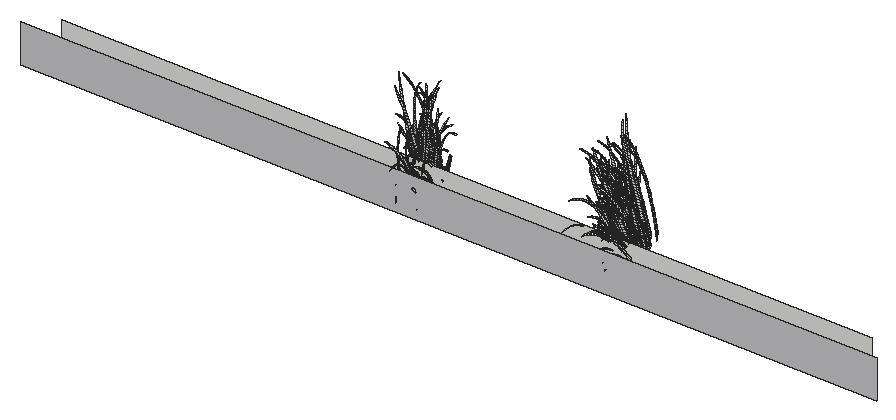
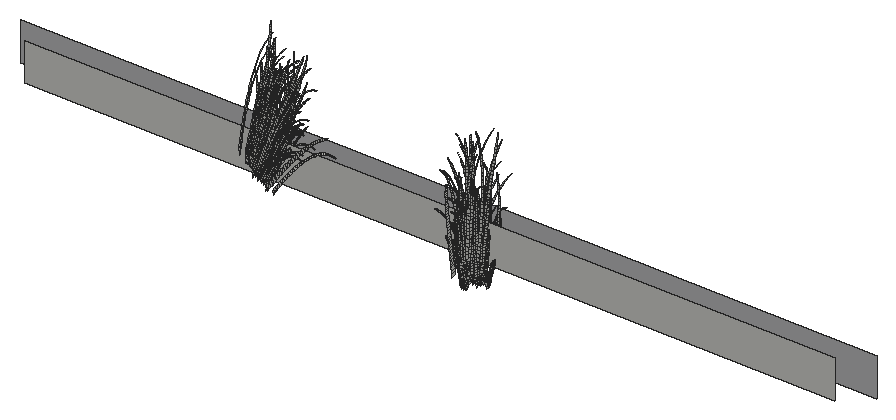
# SketchUp Ruby script. Lengths in inches.
U = 1.inch
M = Sketchup.active_model
def pt(a) = Geom::Point3d.new(a.map { |v| v * U })
def face(e, loops, mat)
  f = e.add_face(loops[0].map { |a| pt(a) })
  loops[1..].each { |l| e.add_face(l.map { |a| pt(a) }).erase! }
  f.material = f.back_material = mat if mat
  f
end
# faces: each face lists its corners as indices into pts; further lists are holes
def faces(e, pts, list, mat = nil) = list.each { |f| face(e, (f[0].is_a?(Array) ? f : [f]).map { |l| l.map { |i| pts[i] } }, mat) }
# xy, xz, yz: faces in a plane at the given z, y or x. An outline is a flat list of corners, or four numbers for a rectangle; further outlines are holes
def ring(l) = l.size == 4 ? [[l[0], l[1]], [l[2], l[1]], [l[2], l[3]], [l[0], l[3]]] : l.each_slice(2).to_a
def flat(e, list, mat, &to3) = list.each { |f| face(e, (f[0].is_a?(Array) ? f : [f]).map { |l| ring(l).map { |u, v| to3.(u, v) } }, mat) }
def xy(e, z, list, mat = nil) = flat(e, list, mat) { |x, y| [x, y, z] }
def xz(e, y, list, mat = nil) = flat(e, list, mat) { |x, z| [x, y, z] }
def yz(e, x, list, mat = nil) = flat(e, list, mat) { |y, z| [x, y, z] }
def lines(e, pts, list) = list.each { |a, b| e.add_line(pt(pts[a]), pt(pts[b])) }
# prism: a flat outline (further loops are holes) pulled along v
def prism(e, loops, v, mat = nil)
  f = face(e, loops, mat); d = Geom::Vector3d.new(v.map { |x| x * U })
  f.pushpull(f.normal.samedirection?(d) ? d.length : -d.length)
end
def box(e, o, s, mat = nil) = prism(e, [[o, [o[0] + s[0], o[1], o[2]], [o[0] + s[0], o[1] + s[1], o[2]], [o[0], o[1] + s[1], o[2]]]], [0, 0, s[2]], mat)
def at(x, y, z, deg = 0) = Geom::Transformation.translation(pt([x, y, z])) * Geom::Transformation.rotation(ORIGIN, Z_AXIS, deg.degrees)
def axes(o, x, y, z) = Geom::Transformation.new([*x, 0, *y, 0, *z, 0, *pt(o).to_a, 1])
def part(name) = M.definitions.add(name)
# library, detail: a bought-in or finely detailed component or shape, given as its bounding box
def library(name, o, s) = part(name).tap { |d| box(d.entities, o, s) }
def detail(e, o, s) = box(e.add_group.entities, o, s)
def put(e, d, t, mat = nil) = e.add_instance(d, t).tap { |i| i.material = mat if mat }
def group(e, t, mat = nil) = e.add_group.tap { |g| g.transformation = t; g.material = mat if mat }.entities
root = M.entities
M.materials.add("[Polished Concrete New]").color = [200, 200, 203]
c1 = part("fur_instance\#8")
p = [[-0.25,1.49,0.03],[0.25,-1.49,-0.03],[0.44,-1.47,1.51],[-0.05,1.47,1.57],[0.65,-1.44,3.05],[0.16,1.45,3.11],
  [0.86,-1.42,4.59],[0.38,1.44,4.65],[1.1,-1.39,6.13],[0.62,1.43,6.18],[1.34,-1.35,7.66],[0.875,1.42,7.72],
  [1.6,-1.32,9.19],[1.14,1.41,9.25],[1.88,-1.28,10.72],[1.43,1.41,10.78],[2.18,-1.24,12.25],[1.73,1.41,12.3],
  [2.49,-1.19,13.77],[2.05,1.41,13.82],[2.83,-1.15,15.29],[2.4,1.41,15.34],[3.18,-1.09,16.8],[2.76,1.42,16.85],
  [3.56,-1.03,18.31],[3.14,1.43,18.35],[3.96,-0.97,19.81],[3.55,1.44,19.85],[4.38,-0.91,21.3],[3.99,1.46,21.35],
  [4.84,-0.83,22.78],[4.45,1.48,22.83],[5.32,-0.76,24.26],[4.93,1.51,24.31],[5.82,-0.67,25.73],[5.45,1.54,25.77],
  [6.36,-0.59,27.18],[6,1.57,27.23],[6.93,-0.49,28.625],[6.58,1.61,28.67],[7.54,-0.39,30.05],[7.19,1.66,30.1],
  [8.18,-0.28,31.47],[7.84,1.71,31.51],[8.85,-0.16,32.86],[8.53,1.77,32.9],[9.57,-0.04,34.24],[9.25,1.83,34.27],
  [10.32,0.09,35.59],[10.02,1.9,35.625],[11.12,0.23,36.92],[10.82,1.97,36.95],[11.95,0.38,38.22],[11.67,2.06,38.25],
  [12.84,0.54,39.49],[12.57,2.14,39.52],[13.76,0.71,40.73],[13.51,2.24,40.76],[14.73,0.89,41.93],[14.49,2.34,41.95],
  [15.75,1.08,43.09],[15.52,2.45,43.11],[16.82,1.28,44.2],[16.6,2.5625,44.23],[17.93,1.5,45.27],[17.73,2.68,45.29],
  [19.08,1.73,46.28],[18.9,2.81,46.3],[20.29,1.97,47.24],[20.125,2.93,47.26],[21.53,2.22,48.13],[21.39,3.0625,48.15],
  [22.82,2.5,48.96],[22.7,3.1875,48.98],[24.14,2.8125,49.72],[24.06,3.3,49.73],[25.48,3.27,50.41]]
faces(c1.entities,p,[[0,1,2,3],[3,2,4,5],[5,4,6,7],[7,6,8,9],[9,8,10,11],[11,10,12,13],[13,12,14,15],[15,14,16,17],
  [17,16,18,19],[19,18,20,21],[21,20,22,23],[23,22,24,25],[25,24,26,27],[27,26,28,29],[29,28,30,31],[31,30,32,33],
  [33,32,34,35],[35,34,36,37],[37,36,38,39],[39,38,40,41],[41,40,42,43],[43,42,44,45],[45,44,46,47],[47,46,48,49],
  [49,48,50,51],[51,50,52,53],[53,52,54,55],[55,54,56,57],[57,56,58,59],[59,58,60,61],[61,60,62,63],[63,62,64,65],
  [65,64,66,67],[67,66,68,69],[69,68,70,71],[71,70,72,73],[73,72,74,75],[75,74,76]])
xz(root,54.02,[[5.25,0,236.6875,10.375]],"[Polished Concrete New]")
xz(root,60.29,[[11.52,0,230.42,10.375]])
put(root,c1,axes([104.88,64.5625,0.37],[-0.10088,0.13062,0.3695],[-0.228,-0.07812,-0.04804],[0.0527,-0.18996,0.43195]))
put(root,c1,axes([102.99,63,-3.69],[0.1143,0.07759,0.29786],[-0.18253,0.04472,0.24081],[0.02462,-0.18668,0.29791]))
put(root,c1,axes([103.16,65.15,0.84],[0.10618,-0.13596,-0.12929],[0.15853,0.08066,0.0353],[0.01505,-0.09183,0.40695]))
put(root,c1,axes([104.26,64.25,-0.45],[-0.04153,-0.12718,-0.27595],[0.20481,-0.00989,-0.14624],[0.04417,-0.15922,0.36205]))
put(root,c1,axes([102.85,63.21,-2.85],[0.19045,-0.03751,-0.06848],[0.03839,0.07261,0.33686],[-0.00736,-0.16676,0.26694]))
put(root,c1,axes([103.43,65.09,0.27],[0.0987,0.11897,0.05521],[-0.14378,0.08662,0.10909],[0.02282,-0.08103,0.37425]))
put(root,c1,axes([103.4,66.72,0.43],[0.11708,-0.12342,-0.00631],[0.12225,0.10057,-0.03033],[0.0076,-0.02912,0.37804]))
put(root,c1,axes([103.375,63.2,-2.95],[0.10158,-0.06914,-0.32205],[0.1701,0.0448,0.14301],[0.02265,-0.17174,0.27406]))
put(root,c1,axes([104.3,63.58,-2.32],[0.00165,-0.10984,-0.26082],[0.18149,0.01453,-0.07449],[0.03836,-0.13829,0.31445]))
put(root,c1,axes([105.61,65.85,1.38],[-0.1604,-0.13739,-0.02167],[0.15059,-0.11716,-0.25101],[0.06963,-0.12643,0.45099]))
put(root,c1,axes([106.29,64.98,0.05],[-0.21667,0.03837,0.29524],[-0.10928,-0.16078,-0.2283],[0.08148,-0.18018,0.43484]))
put(root,c1,axes([103.33,63.9,-1.4],[0.15315,-0.04031,-0.07636],[0.04669,0.1064,0.16007],[0.009,-0.10254,0.31211]))
put(root,c1,axes([105.76,64.41,-1.73],[-0.18644,-0.03104,0.19118],[-0.0143,-0.14214,-0.22961],[0.08573,-0.13206,0.3504]))
put(root,c1,axes([104.09,65.08,0.07],[0.0438,-0.14683,-0.11127],[0.16937,0.03664,-0.05087],[0.03107,-0.07683,0.37846]))
put(root,c1,axes([105.77,67.99,4.57],[-0.20857,-0.13075,0.08955],[0.12369,-0.16885,-0.26752],[0.09431,-0.12712,0.50956]))
put(root,c1,axes([103.61,65.82,-0.01],[0.13914,-0.08385,-0.03496],[0.08075,0.12335,-0.00894],[0.01158,-0.03859,0.35924]))
put(root,c1,axes([105.33,63.78,-3.79],[-0.12758,-0.07753,0.0557],[0.04435,-0.06394,-0.27127],[0.08127,-0.11212,0.2187]))
put(root,c1,axes([105.61,64.0625,-3.08],[-0.14977,-0.06071,0.14936],[0.00439,-0.0935,-0.26844],[0.09015,-0.12438,0.2426]))
put(root,c1,axes([104.98,64.36,-1.99],[-0.08522,-0.11751,-0.02593],[0.11177,-0.04315,-0.23298],[0.08081,-0.09116,0.27707]))
put(root,c1,axes([103.77,63.84,-1.6],[0.12624,-0.07118,-0.14847],[0.09892,0.09301,0.09957],[0.0236,-0.10128,0.3158]))
put(root,c1,axes([103.59,65.81,0.76],[0.11075,-0.11944,-0.11937],[0.13443,0.0987,-0.0216],[0.03784,-0.07056,0.38011]))
put(root,c1,axes([102.82,66.85,4.52],[0.24074,-0.08114,-0.0797],[0.07823,0.19128,0.15934],[0.00596,-0.12377,0.53808]))
put(root,c1,axes([106.61,64.16,-2.25],[-0.23798,-0.07441,0.13592],[0.01899,-0.11962,-0.43721],[0.10286,-0.20447,0.35918]))
put(root,c1,axes([105.24,64.73,-1.81],[-0.09743,0.06774,0.23139],[-0.09599,-0.11967,0.05358],[0.09249,-0.07723,0.28321]))
put(root,c1,axes([104.9,64.89,-0.01],[-0.02184,-0.15888,-0.15748],[0.19236,-0.00034,-0.15603],[0.06127,-0.11125,0.39683]))
put(root,c1,axes([103.6875,65.52,-0.0625],[0.15222,0.03642,-0.07852],[-0.03946,0.13914,0.07531],[0.03898,-0.05711,0.34597]))
put(root,c1,axes([105.6,65.35,-1.97],[-0.11286,0.04976,0.22948],[-0.06771,-0.13658,0.05175],[0.0986,-0.05954,0.28318]))
put(root,c1,axes([104.31,66.85,0.91],[0.07494,-0.15978,-0.03962],[0.16264,0.06715,-0.11216],[0.04856,-0.037,0.39794]))
put(root,c1,axes([105.65,65.16,-0.76],[-0.12334,-0.12969,0.01714],[0.11431,-0.07492,-0.27994],[0.09668,-0.10907,0.33149]))
put(root,c1,axes([104.14,63.32,-2.93],[0.09702,-0.05494,-0.31246],[0.152,0.06601,0.10474],[0.04854,-0.15634,0.25719]))
put(root,c1,axes([105.28,68.49,4.09],[-0.02329,-0.21903,-0.03429],[0.23378,-0.02287,-0.15724],[0.06291,-0.07396,0.52011]))
put(root,c1,axes([104.07,66.1,-0.4],[0.13682,-0.07692,-0.07129],[0.07213,0.1295,-0.07116],[0.03936,-0.02349,0.34277]))
put(root,c1,axes([103.62,63.61,-1.53],[0.22137,0.04305,0.07377],[-0.08148,0.12835,0.33894],[0.02049,-0.18118,0.40078]))
put(root,c1,axes([104.02,63.89,-1.45],[0.16263,0.05278,0.0273],[-0.0671,0.09353,0.2615],[0.03718,-0.13404,0.3048]))
put(root,c1,axes([103.9,66.0625,0.36],[0.1463,-0.07615,-0.10409],[0.07711,0.13848,-0.04067],[0.04559,-0.04329,0.3674]))
put(root,c1,axes([106.05,66.03,-1.21],[-0.14023,0.01888,0.26296],[-0.04453,-0.1614,-0.00292],[0.11023,-0.06656,0.31656]))
put(root,c1,axes([105.92,64.38,-3.03],[-0.13012,-0.10057,0.10963],[0.04873,-0.08061,-0.28847],[0.10836,-0.10823,0.24566]))
put(root,c1,axes([104.49,65.97,-0.32],[0.10839,-0.11453,-0.08174],[0.11795,0.10157,-0.07097],[0.04416,-0.04194,0.35588]))
put(root,c1,axes([104.29,65.1,1.58],[0.14666,-0.13638,-0.25039],[0.18844,0.10867,0.09026],[0.03514,-0.1508,0.47019]))
put(root,c1,axes([106.32,66.26,-1.38],[-0.14894,-0.04461,0.24591],[0.01234,-0.15892,-0.10432],[0.11196,-0.06761,0.32156]))
put(root,c1,axes([105.87,68.4,3.31],[-0.02212,-0.21398,-0.03391],[0.22838,-0.02174,-0.15347],[0.06144,-0.07223,0.50797]))
put(root,c1,axes([103.84,66.9,3.65],[0.23315,0.01342,-0.06471],[-0.02237,0.19719,0.15093],[0.03065,-0.10883,0.50265]))
put(root,c1,axes([104.59,65.17,-0.51],[0.10539,0.11766,-0.04264],[-0.11395,0.08648,0.1779],[0.06944,-0.07112,0.33381]))
put(root,c1,axes([106.53,65.09,-2.05],[-0.10089,0.09227,0.28247],[-0.13958,-0.12254,0.05217],[0.09902,-0.11171,0.33951]))
put(root,c1,axes([105.93,65.4,0.57],[-0.03936,0.14543,0.30601],[-0.20696,-0.07562,0.14027],[0.09659,-0.14879,0.39477]))
put(root,c1,axes([104.2,63.79,-1.64],[0.19476,0.01919,-0.07142],[-0.00771,0.11743,0.2824],[0.0412,-0.14851,0.33769]))
put(root,c1,axes([104.66,68.37,5.28],[0.12423,-0.19532,-0.16493],[0.21975,0.1108,-0.06089],[0.05484,-0.10226,0.55089]))
put(root,c1,axes([104.97,65.86,1.68],[0.10368,0.16194,0.09463],[-0.18699,0.06759,0.22582],[0.06767,-0.12287,0.43828]))
put(root,c1,axes([104.78,63.51,-3.37],[0.10797,-0.02278,-0.25368],[0.09924,0.08349,0.12145],[0.06318,-0.1256,0.22064]))
put(root,c1,axes([104.65,64.28,-1.01],[0.12346,-0.06874,-0.2664],[0.133,0.10274,0.08323],[0.06093,-0.13474,0.32518]))
put(root,c1,axes([105.74,67.7,3.09],[-0.03736,-0.20284,-0.08426],[0.21276,-0.01244,-0.24024],[0.09664,-0.09898,0.46456]))
put(root,c1,axes([104.86,67.38,4.19],[0.143,-0.17445,-0.17187],[0.20045,0.12222,-0.01071],[0.04373,-0.10813,0.53269]))
put(root,c1,axes([104.62,63.54,-2.9],[0.15494,0.00054,-0.15254],[0.03594,0.10834,0.19122],[0.0534,-0.11809,0.285]))
put(root,c1,axes([104.93,65.4,0.34],[0.10826,0.14171,0.01778],[-0.14869,0.07846,0.21324],[0.07154,-0.09642,0.38649]))
put(root,c1,axes([105.6,64.39,-1.4],[0.01148,-0.14011,-0.26001],[0.19146,0.05137,-0.16224],[0.08794,-0.13547,0.35942]))
put(root,c1,axes([105.375,64.33,-2.625],[0.05454,-0.09644,-0.21571],[0.13016,0.08062,-0.0942],[0.08114,-0.09154,0.27821]))
put(root,c1,axes([104.75,68.5,4.97],[0.15717,-0.16888,-0.16909],[0.19008,0.14007,-0.03029],[0.05359,-0.09991,0.53827]))
put(root,c1,axes([106.66,65.53,-1.6875],[-0.06239,0.13265,0.23168],[-0.15342,-0.10065,0.1704],[0.112,-0.09352,0.34293]))
put(root,c1,axes([106.31,67.65,-0.53],[-0.06465,-0.16754,0.157],[0.14103,-0.07728,-0.22676],[0.11827,-0.02606,0.33858]))
put(root,c1,axes([104.48,63.45,-2.45],[0.19478,-0.02841,-0.30734],[0.1247,0.10642,0.29017],[0.06226,-0.20052,0.32988]))
put(root,c1,axes([105.13,63.57,-2.86],[0.10305,-0.05896,-0.3685],[0.16571,0.09891,0.06527],[0.08407,-0.16713,0.29358]))
put(root,c1,axes([104.99,66.04,2.84],[0.19083,0.13184,0.05677],[-0.15811,0.13743,0.27367],[0.05817,-0.15117,0.49659]))
put(root,c1,axes([105.46,65.21,-0.71],[0.13121,0.11551,-0.02739],[-0.11587,0.10209,0.2018],[0.06808,-0.09176,0.36783]))
put(root,c1,axes([105.74,66.79,-2.78],[0.04832,-0.14518,0.00787],[0.12065,0.04323,-0.22286],[0.09094,-0.00311,0.27632]))
put(root,c1,axes([106.59,64.8125,-1.33],[-0.00332,0.15612,0.27725],[-0.2105,-0.04955,0.19049],[0.09652,-0.14869,0.3945]))
put(root,c1,axes([105.71,65.87,-2.31],[0.0496,-0.12974,-0.10453],[0.11629,0.07093,-0.20268],[0.09864,-0.03996,0.27723]))
put(root,c1,axes([106.26,66.11,-3.5],[-0.03175,-0.14429,0.13902],[0.10175,-0.04851,-0.23869],[0.11949,-0.01479,0.22844]))
put(root,c1,axes([106.6,65.14,-2.73],[-0.05491,0.09737,0.28251],[-0.12379,-0.11722,0.16383],[0.12913,-0.0934,0.26231]))
put(root,c1,axes([106.8,65.13,-2.91],[-0.0662,0.08995,0.30205],[-0.12202,-0.12772,0.14438],[0.13238,-0.09575,0.2689]))
put(root,c1,axes([107.73,65.6,-1.92],[-0.14869,0.01051,0.38769],[-0.10168,-0.16677,-0.09879],[0.14048,-0.14032,0.31849]))
put(root,c1,axes([105.58,64.83,-2.4],[0.12216,0.08749,-0.1288],[-0.05725,0.10364,0.19567],[0.09123,-0.07618,0.27934]))
put(root,c1,axes([106.86,65.27,-2.83],[-0.06626,-0.1567,-0.04431],[0.12258,-0.00555,-0.33309],[0.13287,-0.09611,0.2699]))
put(root,c1,axes([107.13,66.85,-3.31],[-0.09134,-0.12785,0.22656],[0.07697,-0.11104,-0.22116],[0.1384,-0.04262,0.25929]))
put(root,c1,axes([106.32,64.43,-2.49],[0.07572,0.13089,0.20219],[-0.15985,-0.01369,0.30106],[0.10643,-0.14683,0.2864]))
put(root,c1,axes([105.71,66.13,-0.12],[0.16409,-0.04331,-0.20606],[0.05728,0.16704,-0.00737],[0.08461,-0.06565,0.38043]))
put(root,c1,axes([106.12,66.375,-3.28],[0.06266,-0.1249,-0.10853],[0.0861,0.08678,-0.25374],[0.11938,-0.01478,0.22823]))
put(root,c1,axes([105.9,64.99,-2.2],[0.14109,0.00407,-0.23949],[0.03377,0.14579,0.07817],[0.0981,-0.08192,0.30039]))
put(root,c1,axes([106.16,65.55,-1.62],[0.12005,-0.06141,-0.26447],[0.09556,0.14151,-0.0324],[0.10376,-0.08664,0.31771]))
put(root,c1,axes([106.03,64.79,-1.98],[0.16454,0.02683,-0.22071],[0.01929,0.1451,0.16624],[0.09525,-0.10745,0.32659]))
put(root,c1,axes([108.56,65.3,-3.34],[-0.15559,-0.16713,0.03304],[0.11706,-0.06849,-0.43118],[0.15185,-0.15167,0.34426]))
put(root,c1,axes([106.49,66.41,-3.37],[0.068,-0.12804,-0.12081],[0.08818,0.09434,-0.26208],[0.12484,-0.01545,0.23865]))
put(root,c1,axes([105.9375,66.45,1.42],[0.20769,0.04966,-0.15926],[-0.03101,0.17814,0.18526],[0.08167,-0.11008,0.44127]))
put(root,c1,axes([106.53,65.6,-2.96],[0.06859,-0.09014,-0.25373],[0.09618,0.12505,-0.16822],[0.12923,-0.06487,0.24688]))
put(root,c1,axes([106.05,64.54,-0.8],[0.20792,-0.04098,-0.29203],[0.11115,0.15527,0.21492],[0.07916,-0.17504,0.42246]))
put(root,c1,axes([106.57,65.61,-2.41],[0.12063,-0.06515,-0.25144],[0.08341,0.14829,-0.07405],[0.10987,-0.06634,0.31554]))
put(root,c1,axes([106.75,65.05,-0.75],[0.15805,0.15051,0.05502],[-0.15454,0.08321,0.34889],[0.10135,-0.15612,0.41421]))
put(root,c1,axes([106.875,67.2,1.77],[0.20327,-0.05604,-0.25675],[0.08292,0.19878,0.03195],[0.09822,-0.10059,0.47212]))
put(root,c1,axes([108.15,64.87,-3.34],[0.10396,-0.07911,-0.43973],[0.18772,0.13868,-0.01375],[0.12911,-0.17813,0.34745]))
put(root,c1,axes([108.54,67.78,-0.56],[0.04979,-0.1895,-0.18773],[0.18438,0.09265,-0.2851],[0.14308,-0.0864,0.41092]))
put(root,c1,axes([107.64,64.82,-3.64],[0.1674,0.12348,-0.15342],[-0.05527,0.10723,0.36025],[0.13749,-0.13733,0.3117]))
put(root,c1,axes([158.09,68.76,3.75],[-0.02161,-0.16628,-0.28389],[0.16425,-0.14433,0.32408],[-0.18224,-0.08282,0.344]))
put(root,c1,axes([158.15,66.78,1.77],[-0.07933,-0.07892,-0.44402],[0.19255,-0.17562,0.06989],[-0.14788,-0.14983,0.35337]))
put(root,c1,axes([160.83,67.33,7.77],[-0.23554,0.05296,-0.19778],[0.0198,-0.2043,-0.19606],[-0.09324,-0.11985,0.49597]))
put(root,c1,axes([160.625,68.95,7.54],[-0.04128,-0.19919,-0.10991],[0.2038,-0.09544,0.23105],[-0.11682,-0.05581,0.46862]))
put(root,c1,axes([159.8,67.08,2],[0.13283,-0.0342,0.36955],[-0.05695,0.18902,0.06859],[-0.15898,-0.07225,0.3001]))
put(root,c1,axes([162.76,64.83,2.51],[-0.12873,0.10197,-0.18861],[-0.01018,-0.10343,-0.24101],[-0.11719,-0.08155,0.24232]))
put(root,c1,axes([162.04,68.05,6.68],[-0.08516,-0.14739,-0.15062],[0.16457,-0.13044,0.17116],[-0.1041,-0.04973,0.41758]))
put(root,c1,axes([162.85,64.22,2.92],[-0.15935,0.03269,-0.28558],[0.09029,-0.13292,-0.22683],[-0.09601,-0.14239,0.28508]))
put(root,c1,axes([162.85,64.65,2.21],[-0.14081,0.09765,-0.1356],[-0.01218,-0.08683,-0.27326],[-0.10036,-0.10168,0.23982]))
put(root,c1,axes([163,66.09,6.5],[-0.18347,0.1171,-0.07334],[-0.07461,-0.13251,-0.22152],[-0.07812,-0.10043,0.41558]))
put(root,c1,axes([162.88,64.51,2.71],[-0.15082,0.11254,-0.07354],[-0.05779,-0.09193,-0.25822],[-0.08893,-0.09949,0.31347]))
put(root,c1,axes([162.86,66.52,5.94],[-0.149,-0.04647,-0.21352],[0.09287,-0.17245,0.02054],[-0.09229,-0.06322,0.38876]))
put(root,c1,axes([162.38,64.27,3.03],[-0.09966,0.12678,0.30336],[-0.19172,0.0268,-0.26785],[-0.07616,-0.17634,0.31506]))
put(root,c1,axes([161.625,66.42,3.22],[0.05365,-0.16969,-0.03778],[0.13986,-0.00916,0.27148],[-0.1167,-0.06341,0.32492]))
put(root,c1,axes([163.08,64.77,2.88],[-0.10552,0.13111,0.03774],[-0.1075,-0.03434,-0.24755],[-0.08294,-0.09279,0.29236]))
put(root,c1,axes([163.64,64.85,6.41],[-0.23362,0.09843,0.07428],[-0.08627,-0.11761,-0.36241],[-0.04076,-0.18596,0.42692]))
put(root,c1,axes([162.83,65.09,2.59],[-0.05906,0.14196,0.06951],[-0.12604,0.00717,-0.23329],[-0.09379,-0.07416,0.28621]))
put(root,c1,axes([161.53,65.05,1.76],[0.08197,-0.14846,-0.17255],[0.1435,-0.03613,0.3122],[-0.11735,-0.1189,0.28043]))
put(root,c1,axes([163.66,67.41,9.42],[-0.2227,-0.02851,-0.13015],[0.07795,-0.20389,-0.10631],[-0.04666,-0.10194,0.51151]))
put(root,c1,axes([163.05,65.87,2.94],[-0.05395,-0.10392,-0.15053],[0.10796,-0.10426,0.17042],[-0.10255,-0.03484,0.272]))
put(root,c1,axes([163.64,64.13,3.64],[-0.17727,0.00029,-0.20455],[0.08516,-0.1353,-0.21935],[-0.05731,-0.14134,0.34686]))
put(root,c1,axes([163.39,64.61,3.51],[-0.10062,-0.049,-0.26041],[0.12035,-0.13237,-0.01381],[-0.08638,-0.09663,0.30447]))
put(root,c1,axes([163.7,66.22,4.12],[-0.12457,-0.03797,-0.15408],[0.05979,-0.14532,0.07008],[-0.07901,-0.02356,0.31353]))
put(root,c1,axes([163.34,64.01,4.09],[-0.15374,0.14658,0.25603],[-0.19784,-0.04817,-0.27014],[-0.04101,-0.18709,0.42951]))
put(root,c1,axes([161.73,65.41,1.76],[0.13307,-0.06357,0.27984],[-0.03809,0.14212,0.17121],[-0.12562,-0.08741,0.25976]))
put(root,c1,axes([163.61,64.3,2.375],[-0.0986,0.1202,0.03133],[-0.09749,-0.03341,-0.22837],[-0.07635,-0.08541,0.26912]))
put(root,c1,axes([163.4,64.0625,1.98],[-0.08725,-0.02366,-0.29756],[0.12591,-0.11202,-0.06714],[-0.0803,-0.1191,0.23844]))
put(root,c1,axes([163.93,64.14,2.95],[-0.15103,0.03829,-0.1475],[0.02836,-0.11444,-0.19385],[-0.06472,-0.10394,0.28282]))
put(root,c1,axes([161.23,65.9,3.56],[0.17403,-0.06722,0.24815],[-0.01797,0.16553,0.179],[-0.11789,-0.09322,0.35975]))
put(root,c1,axes([162.9,63.5625,1.96],[-0.07738,0.12181,0.42116],[-0.24475,0.02807,-0.19007],[-0.04925,-0.2161,0.35893]))
put(root,c1,axes([164.11,63.58,2.95],[-0.19758,0.0885,0.1271],[-0.09447,-0.05952,-0.37318],[-0.04202,-0.18438,0.30623]))
put(root,c1,axes([162.6,65.45,3.43],[0.04667,0.10587,0.22641],[-0.14224,0.11026,-0.13144],[-0.10087,-0.07976,0.30781]))
put(root,c1,axes([163.49,65,6.18],[-0.12023,0.16893,0.15811],[-0.19192,-0.04724,-0.20175],[-0.05017,-0.13536,0.45159]))
put(root,c1,axes([163.75,64.82,4.52],[-0.1513,-0.02821,-0.17374],[0.08683,-0.1419,-0.10144],[-0.05423,-0.09755,0.35603]))
put(root,c1,axes([163.87,64.62,3.44],[-0.07947,0.12548,0.07397],[-0.11521,-0.01055,-0.22059],[-0.07706,-0.08621,0.27164]))
put(root,c1,axes([163.58,66.85,3.86],[-0.06439,-0.12354,-0.04587],[0.12333,-0.08786,0.16125],[-0.07712,-0.0102,0.31415]))
put(root,c1,axes([163.03,65.11,2.49],[0.02731,-0.14018,-0.06519],[0.12315,-0.02871,0.2214],[-0.09827,-0.0534,0.27359]))
put(root,c1,axes([162.42,64.66,1.89],[0.09631,-0.13966,-0.10726],[0.11682,-0.00954,0.30869],[-0.10751,-0.10893,0.25692]))
put(root,c1,axes([164.35,64.74,5.09],[-0.18173,0.02045,-0.09763],[0.0261,-0.14072,-0.18343],[-0.04068,-0.10974,0.36609]))
put(root,c1,axes([162.83,65.89,3.28],[0.06905,-0.15041,0.07394],[0.1069,0.0384,0.22809],[-0.10814,-0.03674,0.28683]))
put(root,c1,axes([162.8,66.28,4.85],[0.02994,-0.16585,-0.05499],[0.16129,-0.01842,0.19273],[-0.08623,-0.05907,0.36324]))
put(root,c1,axes([164.4375,63.5,2.53],[-0.18497,0.04944,-0.02341],[-0.00878,-0.07542,-0.33252],[-0.03553,-0.1559,0.25894]))
put(root,c1,axes([164.15,65.75,5.45],[-0.14413,-0.05167,-0.11933],[0.08701,-0.14734,-0.01287],[-0.04763,-0.0596,0.37283]))
put(root,c1,axes([163.87,63.85,2.15],[-0.04193,0.09854,0.23039],[-0.14173,0.04993,-0.18317],[-0.07748,-0.11492,0.23007]))
put(root,c1,axes([163.63,66.04,4.19],[-0.02354,-0.13666,-0.06934],[0.13862,-0.06024,0.1585],[-0.07899,-0.03774,0.31687]))
put(root,c1,axes([164.59,63.625,2.59],[-0.15528,0.03655,-0.09389],[0.01601,-0.10098,-0.21878],[-0.04549,-0.11219,0.27533]))
put(root,c1,axes([164.625,64.46,4.13],[-0.15238,0.03287,-0.097],[0.00948,-0.12228,-0.14695],[-0.04746,-0.08538,0.3116]))
put(root,c1,axes([163.87,65.7,4.59],[-0.02967,-0.13006,-0.11002],[0.14258,-0.07093,0.13984],[-0.07655,-0.05244,0.32247]))
put(root,c1,axes([162.75,65.01,2.95],[0.10962,-0.14134,0.02858],[0.09848,0.05163,0.25611],[-0.09929,-0.07851,0.30299]))
put(root,c1,axes([164.24,65.02,5.3],[-0.07622,0.14548,0.11566],[-0.15943,-0.01772,-0.1678],[-0.05494,-0.09882,0.36066]))
put(root,c1,axes([164.96,65.69,8.0625],[-0.23536,0.00031,-0.04255],[0.03502,-0.16941,-0.26023],[-0.00865,-0.15175,0.46324]))
put(root,c1,axes([163.34,63.92,2.05],[0.07176,0.04443,0.32956],[-0.1495,0.11571,0.02095],[-0.08693,-0.12893,0.25813]))
put(root,c1,axes([164.49,67.92,8.8],[-0.16552,-0.11118,-0.05649],[0.14207,-0.16762,-0.00154],[-0.02412,-0.05905,0.48802]))
put(root,c1,axes([164.45,63.68,3.4],[-0.1192,0.12425,0.22535],[-0.17166,-0.03356,-0.21354],[-0.0342,-0.15606,0.35826]))
put(root,c1,axes([164.16,65.45,4.62],[-0.02927,-0.12714,-0.10789],[0.13946,-0.06963,0.13664],[-0.0749,-0.05131,0.31553]))
put(root,c1,axes([162.41,64.84,4.17],[0.13498,-0.15634,-0.12045],[0.15269,0.03421,0.29976],[-0.08583,-0.13785,0.37509]))
put(root,c1,axes([163.65,66.07,7.93],[-0.00008,0.17023,0.2439],[-0.22913,0.05018,-0.08813],[-0.05076,-0.13695,0.4569]))
put(root,c1,axes([162.48,66.21,5.49],[0.15632,-0.13539,0.07566],[0.09629,0.11232,0.20743],[-0.0859,-0.08088,0.3964]))
put(root,c1,axes([162.37,63.875,2.16],[0.17581,0.00429,0.35889],[-0.15371,0.13999,0.25001],[-0.08231,-0.1906,0.34052]))
put(root,c1,axes([163.56,65.44,6.28],[0.05112,0.14176,0.22694],[-0.19757,0.09246,-0.06236],[-0.06344,-0.11412,0.4165]))
put(root,c1,axes([163.9,65.46,4.97],[0.0229,-0.1484,-0.09458],[0.15576,-0.02704,0.16403],[-0.07366,-0.06935,0.33993]))
put(root,c1,axes([164.18,67.02,7.98],[-0.04613,-0.168,-0.12838],[0.20048,-0.07761,0.07112],[-0.05022,-0.08162,0.45074]))
put(root,c1,axes([163.7,66.9375,7.05],[0.01336,-0.18156,-0.05149],[0.1916,-0.02315,0.12623],[-0.05991,-0.05859,0.42926]))
put(root,c1,axes([163.25,65.12,3.3125],[0.13306,-0.03251,0.2141],[-0.03468,0.1366,0.1095],[-0.09265,-0.07326,0.28274]))
put(root,c1,axes([164.75,65.3,6.55],[-0.14651,-0.09517,-0.11625],[0.13838,-0.13795,-0.08263],[-0.01824,-0.0963,0.42995]))
put(root,c1,axes([165.47,66.82,9.01],[-0.22374,-0.02944,-0.01516],[0.05551,-0.18692,-0.16154],[0.00543,-0.11272,0.49003]))
put(root,c1,axes([164.37,63.75,3.09],[-0.00857,-0.10681,-0.26092],[0.17656,-0.05814,0.06779],[-0.05152,-0.12704,0.31177]))
put(root,c1,axes([163.27,64.66,3.74],[0.14194,0.01295,0.23971],[-0.09799,0.13483,0.13149],[-0.07264,-0.11667,0.31745]))
put(root,c1,axes([164.13,64.1875,3.29],[0.04246,-0.11664,-0.17724],[0.14637,-0.02684,0.16417],[-0.06419,-0.10309,0.2805]))
put(root,c1,axes([165.28,66.82,7.26],[-0.13872,-0.10688,-0.05008],[0.13478,-0.14007,-0.01499],[-0.01621,-0.05768,0.43132]))
put(root,c1,axes([164.92,67.18,7.01],[-0.09202,-0.14419,-0.02135],[0.16494,-0.10399,0.03603],[-0.02333,-0.03794,0.42396]))
put(root,c1,axes([164.1,66.01,4.62],[0.09225,-0.12894,0.11038],[0.10291,0.0771,0.12838],[-0.07903,-0.02356,0.31361]))
put(root,c1,axes([164.24,63.42,1.75],[0.04168,-0.09258,-0.28201],[0.16554,-0.04371,0.15063],[-0.06017,-0.13932,0.24891]))
put(root,c1,axes([163.4,64.72,3.96],[0.15549,-0.01208,0.20833],[-0.06905,0.13306,0.17126],[-0.07165,-0.11508,0.31313]))
put(root,c1,axes([165.78,65.93,7.09],[-0.18618,-0.03996,-0.02577],[0.06509,-0.15689,-0.1364],[0.00464,-0.09644,0.41925]))
put(root,c1,axes([165.79,65.55,5.67],[-0.15853,0.06077,0.01255],[-0.05151,-0.13731,-0.04414],[-0.00488,-0.05314,0.37046]))
put(root,c1,axes([166.21,64.09,5.28],[-0.25079,-0.01126,0.01167],[0.02691,-0.14432,-0.37072],[0.02191,-0.19373,0.42855]))
put(root,c1,axes([165.67,63.75,3.77],[-0.15193,-0.01941,-0.09588],[0.0644,-0.09304,-0.22233],[-0.00624,-0.12588,0.27933]))
put(root,c1,axes([165.97,62.98,1.5],[-0.16406,0.03446,0.0684],[-0.03839,-0.06194,-0.29017],[-0.00638,-0.14462,0.2315]))
put(root,c1,axes([163.07,63.98,2.34],[0.18766,-0.05407,0.15304],[-0.0375,0.10124,0.3241],[-0.06745,-0.15619,0.27904]))
put(root,c1,axes([164.77,65.78,8.46],[-0.04308,0.17847,0.273],[-0.24701,-0.00413,-0.05166],[-0.00912,-0.15991,0.48813]))
put(root,c1,axes([164.14,64.11,4.21],[0.03417,-0.12525,-0.29157],[0.20378,-0.0224,0.09589],[-0.03382,-0.15429,0.3542]))
put(root,c1,axes([164.43,64.54,5.55],[0.00591,-0.15376,-0.2335],[0.21361,-0.03099,0.04882],[-0.02765,-0.13326,0.41924]))
put(root,c1,axes([165.23,64.44,5.5],[-0.06192,0.14505,0.21697],[-0.19671,-0.02273,-0.07174],[-0.0075,-0.13152,0.40147]))
put(root,c1,axes([166.47,63.75,4.18],[-0.22603,-0.01056,0.00948],[0.02497,-0.13008,-0.33426],[0.01976,-0.17466,0.38636]))
put(root,c1,axes([164.99,65.36,6.98],[0.0038,0.14954,0.23139],[-0.20994,0.03733,-0.03743],[-0.02717,-0.13094,0.41195]))
put(root,c1,axes([165.09,65.625,5.18],[-0.04654,-0.13259,-0.03011],[0.14978,-0.05997,0.02545],[-0.01873,-0.03986,0.3514]))
put(root,c1,axes([165.13,63.08,1.48],[-0.02123,-0.06781,-0.31584],[0.17417,-0.05199,-0.00113],[-0.03366,-0.14772,0.24534]))
put(root,c1,axes([166.01,64.51,6.24],[-0.18897,-0.07724,-0.16578],[0.14014,-0.11074,-0.30364],[0.02044,-0.18069,0.39971]))
put(root,c1,axes([165.16,65.26,6.49],[-0.0211,0.16438,0.13367],[-0.19675,0.00758,-0.04177],[-0.01791,-0.09455,0.42215]))
put(root,c1,axes([165.83,66.02,6.79],[-0.1296,-0.11177,-0.03307],[0.13714,-0.12794,-0.0397],[-0.00189,-0.06022,0.41924]))
put(root,c1,axes([164.66,63.68,2.85],[0.0606,-0.10906,-0.18612],[0.14677,-0.00638,0.15494],[-0.04628,-0.11412,0.28007]))
put(root,c1,axes([166.25,65.31,7.4],[-0.15736,0.12863,0.21317],[-0.17096,-0.10355,-0.14422],[0.01307,-0.14881,0.45294]))
put(root,c1,axes([166.19,64.49,5.2],[-0.16225,-0.04777,-0.05886],[0.07812,-0.11873,-0.19059],[0.01013,-0.11533,0.35104]))
put(root,c1,axes([166.02,65.42,6.21],[-0.13495,-0.09194,-0.07228],[0.12419,-0.11921,-0.10694],[0.00432,-0.08968,0.38985]))
put(root,c1,axes([165.16,66.05,6.99],[-0.00432,-0.15952,-0.128],[0.19173,-0.03266,0.04648],[-0.02798,-0.08806,0.41192]))
put(root,c1,axes([164.6875,63.94,3.66],[0.10535,0.0488,0.23666],[-0.12967,0.10407,0.09442],[-0.04869,-0.12008,0.29468]))
put(root,c1,axes([165.16,66.96,6.43],[-0.00822,-0.16722,0.01164],[0.17876,-0.02595,0.03382],[-0.01925,-0.0303,0.40131]))
put(root,c1,axes([166.3,64.4,4.66],[-0.14242,0.06423,0.07833],[-0.06984,-0.11466,-0.07925],[0.01251,-0.07634,0.33832]))
put(root,c1,axes([166.35,64.98,6.03],[-0.1422,0.11091,0.11586],[-0.12628,-0.11191,-0.06649],[0.015,-0.09153,0.40561]))
put(root,c1,axes([166.61,67.46,8.36],[-0.17633,-0.09809,0.01724],[0.1199,-0.16919,-0.04915],[0.01352,-0.05835,0.47546]))
put(root,c1,axes([166.38,63.61,3.54],[-0.13701,0.06738,0.19305],[-0.11347,-0.07671,-0.17654],[0.01546,-0.13663,0.30225]))
put(root,c1,axes([166.36,65.19,5.49],[-0.14765,0.06695,0.09599],[-0.07527,-0.12279,-0.06548],[0.02169,-0.07701,0.35566]))
put(root,c1,axes([166.73,67.52,9.43],[-0.22223,-0.05187,0.06437],[0.06185,-0.19269,-0.14793],[0.04097,-0.1013,0.49904]))
put(root,c1,axes([164.36,66.37,5.93],[0.1666,-0.05285,0.10887],[0.0248,0.15525,0.04679],[-0.05548,-0.04238,0.37888]))
